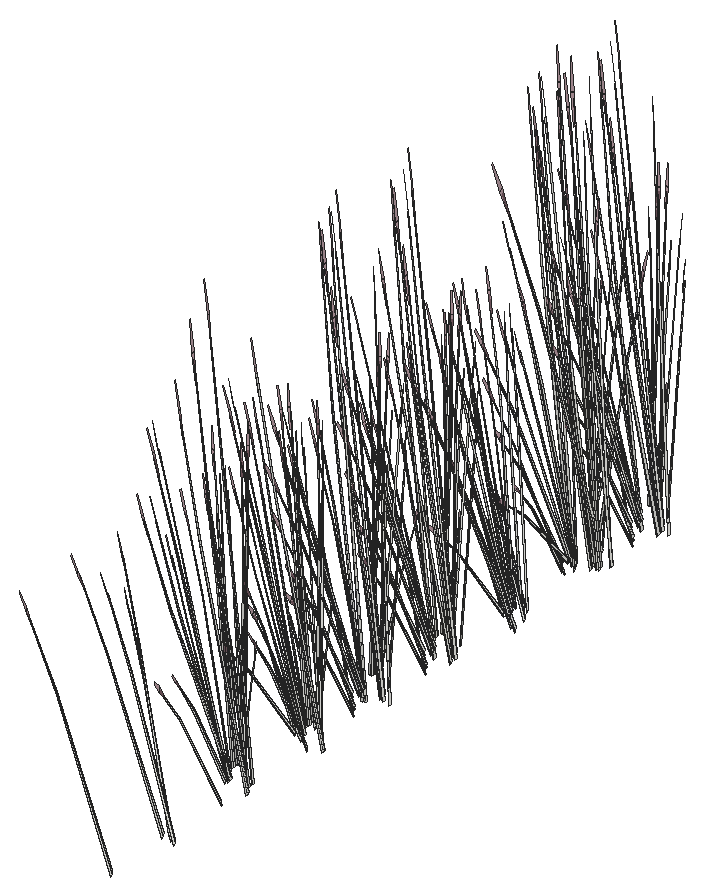
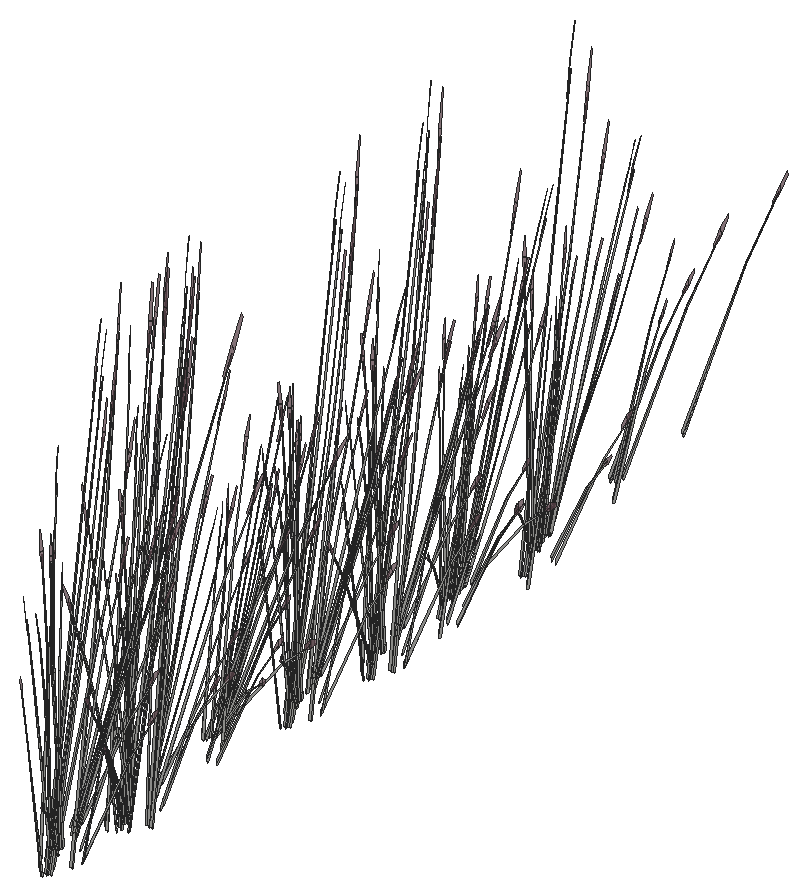
# SketchUp Ruby script. Lengths in inches.
U = 1.inch
M = Sketchup.active_model
def pt(a) = Geom::Point3d.new(a.map { |v| v * U })
def face(e, loops, mat)
  f = e.add_face(loops[0].map { |a| pt(a) })
  loops[1..].each { |l| e.add_face(l.map { |a| pt(a) }).erase! }
  f.material = f.back_material = mat if mat
  f
end
# faces: each face lists its corners as indices into pts; further lists are holes
def faces(e, pts, list, mat = nil) = list.each { |f| face(e, (f[0].is_a?(Array) ? f : [f]).map { |l| l.map { |i| pts[i] } }, mat) }
# xy, xz, yz: faces in a plane at the given z, y or x. An outline is a flat list of corners, or four numbers for a rectangle; further outlines are holes
def ring(l) = l.size == 4 ? [[l[0], l[1]], [l[2], l[1]], [l[2], l[3]], [l[0], l[3]]] : l.each_slice(2).to_a
def flat(e, list, mat, &to3) = list.each { |f| face(e, (f[0].is_a?(Array) ? f : [f]).map { |l| ring(l).map { |u, v| to3.(u, v) } }, mat) }
def xy(e, z, list, mat = nil) = flat(e, list, mat) { |x, y| [x, y, z] }
def xz(e, y, list, mat = nil) = flat(e, list, mat) { |x, z| [x, y, z] }
def yz(e, x, list, mat = nil) = flat(e, list, mat) { |y, z| [x, y, z] }
def lines(e, pts, list) = list.each { |a, b| e.add_line(pt(pts[a]), pt(pts[b])) }
# prism: a flat outline (further loops are holes) pulled along v
def prism(e, loops, v, mat = nil)
  f = face(e, loops, mat); d = Geom::Vector3d.new(v.map { |x| x * U })
  f.pushpull(f.normal.samedirection?(d) ? d.length : -d.length)
end
def box(e, o, s, mat = nil) = prism(e, [[o, [o[0] + s[0], o[1], o[2]], [o[0] + s[0], o[1] + s[1], o[2]], [o[0], o[1] + s[1], o[2]]]], [0, 0, s[2]], mat)
def at(x, y, z, deg = 0) = Geom::Transformation.translation(pt([x, y, z])) * Geom::Transformation.rotation(ORIGIN, Z_AXIS, deg.degrees)
def axes(o, x, y, z) = Geom::Transformation.new([*x, 0, *y, 0, *z, 0, *pt(o).to_a, 1])
def part(name) = M.definitions.add(name)
# library, detail: a bought-in or finely detailed component or shape, given as its bounding box
def library(name, o, s) = part(name).tap { |d| box(d.entities, o, s) }
def detail(e, o, s) = box(e.add_group.entities, o, s)
def put(e, d, t, mat = nil) = e.add_instance(d, t).tap { |i| i.material = mat if mat }
def group(e, t, mat = nil) = e.add_group.tap { |g| g.transformation = t; g.material = mat if mat }.entities
root = M.entities
M.materials.add("LightPink_Translucent").color = [144, 107, 117]
M.materials["LightPink_Translucent"].alpha = 0.75
c1 = part("blade")
p = [[2.15,0.21,22],[0,0.17,0],[0.09,0.45,0],[2.18,0.31,22],[2.29,0.31,22],[0.38,0.45,0],
  [2.48,0.24,33],[2.49,0.24,33],[2.48,0.22,33]]
faces(c1.entities,p,[[0,1,2,3],[4,5,2,3],[6,3,4,7],[8,0,3,6]])
c2 = part("seeds")
p = [[0.3,-0.1,1.38],[-0.01,-0.03,1.59],[-0.01,-0.03,0.03],[0.14,-0.07,-0.07],[0.29,-0.03,3],[0.15,0.01,3.11]]
faces(c2.entities,p,[[0,1,2,3],[1,0,4,5]],"LightPink_Translucent")
c3 = part("blade with seeds")
put(c3.entities,c1,at(0,0,0))
put(c3.entities,c2,axes([2.4,0.25,30.99],[1.5799,-0.05474,1.17369],[-0.12525,1.92788,0.29478],[-0.07173,-0.02425,1.56792]))
put(root,c3,axes([401.41,385.93,-7.3],[0.42502,0.15163,0.32977],[-0.12396,0.44238,-0.42575],[-0.17112,0.04056,0.81462]))
put(root,c3,axes([402.65,354.11,-8.39],[0.12773,-0.16701,1.59586],[0.32252,0.4508,0.12904],[-0.22121,0.20529,0.68222]))
put(root,c3,axes([402.3,364.67,-10.61],[0.01297,0.08566,1.6421],[-0.26146,0.44735,-0.25086],[-0.18572,-0.02255,0.2797]))
put(root,c3,axes([401.6,374.12,-7.3],[0.29098,0.34031,0.32977],[-0.33226,0.32215,-0.42575],[-0.16881,-0.04902,0.81462]))
put(root,c3,axes([401.49,417.08,-7.6],[0.02575,-0.41332,0.05988],[0.38885,0.01133,0.47138],[-0.14895,-0.04325,0.71878]))
put(root,c3,axes([401.88,354.55,-7.78],[-0.44516,0.07768,-0.32977],[-0.11755,-0.44407,0.42575],[-0.12757,0.11927,0.81462]))
put(root,c3,axes([400.57,420.61,-7.61],[-0.01271,0.10756,1.62908],[0.36076,0.37419,-0.25764],[-0.09444,0.17695,0.13065]))
put(root,c3,axes([402.39,373.52,-7.36],[-0.43608,-0.26272,-0.66157],[0.30991,-0.46038,0.07984],[-0.158,-0.15687,0.93586]))
put(root,c3,axes([402.59,419.37,-10.08],[-0.53199,-0.08911,-0.58063],[0.11226,-0.54969,-0.15239],[-0.15876,-0.06661,1.28164]))
put(root,c3,axes([402.68,416.37,-6.94],[-0.34131,0.52108,-0.12682],[-0.49429,-0.3002,-0.70393],[-0.17182,-0.14722,1.06961]))
put(root,c3,axes([401.6,405.53,-7.62],[-0.00954,0.06515,1.65179],[-0.47055,0.23645,-0.15608],[-0.13847,-0.12087,0.29231]))
put(root,c3,axes([402.18,373.53,-7.64],[-0.50465,0.12921,-0.47583],[-0.08828,-0.48932,-0.36857],[-0.13555,-0.14022,0.91046]))
put(root,c3,axes([401.48,387.31,-7.64],[0.13138,0.49631,-0.47583],[-0.49754,0.08682,-0.36857],[-0.14258,0.13331,0.91046]))
put(root,c3,axes([401.64,355.87,-10.61],[0.0686,0.0543,1.6421],[0.11632,0.50315,-0.25086],[-0.15204,0.10729,0.2797]))
put(root,c3,axes([402.37,362.625,-7.62],[0.03791,0.05424,1.65179],[-0.18278,0.48761,-0.15608],[-0.18511,0.00353,0.29231]))
put(root,c3,axes([401.62,384.67,-7.6],[0.02575,-0.41332,0.05988],[0.38885,0.01133,0.47138],[-0.14895,-0.04325,0.71878]))
put(root,c3,axes([401.1,406.47,-9.59],[-0.03097,0.17781,1.33163],[-0.45273,0.14885,-0.28638],[-0.10583,-0.22982,0.56934]))
put(root,c3,axes([401.75,417.39,-7.3],[0.29098,0.34031,0.32977],[-0.33226,0.32215,-0.42575],[-0.16881,-0.04902,0.81462]))
put(root,c3,axes([400.7,388.2,-7.61],[-0.01271,0.10756,1.62908],[0.36076,0.37419,-0.25764],[-0.09444,0.17695,0.13065]))
put(root,c3,axes([401.54,352.91,-9.42],[0.3265,-0.03889,1.06958],[-0.20711,0.3427,0.78586],[-0.16135,-0.05141,0.23558]))
put(root,c3,axes([404.56,395.59,-8.89],[0.14537,-0.07863,1.64882],[0.05013,0.549,0.12904],[-0.31487,0.07285,0.5893]))
put(root,c3,axes([401.24,406.93,-8.39],[0.1169,0.17452,1.59586],[-0.54019,0.14692,0.12904],[-0.12209,-0.27397,0.68222]))
put(root,c3,axes([402.72,386.95,-10.08],[-0.53199,-0.08911,-0.58063],[0.11226,-0.54969,-0.15239],[-0.15876,-0.06661,1.28164]))
put(root,c3,axes([402.53,416.79,-7.36],[-0.43608,-0.26272,-0.66157],[0.30991,-0.46038,0.07984],[-0.158,-0.15687,0.93586]))
put(root,c3,axes([402.82,383.95,-6.94],[-0.34131,0.52108,-0.12682],[-0.49429,-0.3002,-0.70393],[-0.17182,-0.14722,1.06961]))
put(root,c3,axes([402.24,409.85,-9.52],[-0.51635,0.36087,-0.27094],[-0.34336,-0.5099,-0.46562],[-0.1274,-0.05178,1.4872]))
put(root,c3,axes([402.33,416.8,-7.64],[-0.50465,0.12921,-0.47583],[-0.08828,-0.48932,-0.36857],[-0.13555,-0.14022,0.91046]))
put(root,c3,axes([401.6,366.82,-9.42],[0.21313,-0.24635,1.06958],[0.0841,0.38999,0.78586],[-0.15402,0.06983,0.23558]))
put(root,c3,axes([401.74,377.13,-10.12],[-0.47863,-0.27177,-0.46235],[0.28609,-0.48733,0],[-0.10901,-0.0619,1.46668]))
put(root,c3,axes([400.8125,410.98,-7.59],[-0.36417,-0.37086,0.447],[0.38674,-0.31985,0.36857],[-0.06718,0.174,0.92496]))
put(root,c3,axes([401.53,373.08,-10.61],[-0.04954,0.0716,1.6421],[-0.50062,0.15438,-0.25086],[-0.12094,-0.14044,0.2797]))
put(root,c3,axes([400.97,376.09,-7.3125],[0.47307,0.29971,-0.11324],[-0.27254,0.43404,-0.62851],[-0.13365,0.15087,0.95501]))
put(root,c3,axes([402.79,362.3,-7.61],[-0.11004,-0.00384,1.62908],[-0.35032,0.38367,-0.25764],[-0.18692,-0.07839,0.13065]))
put(root,c3,axes([401.88,384.98,-7.3],[0.29098,0.34031,0.32977],[-0.33226,0.32215,-0.42575],[-0.16881,-0.04902,0.81462]))
put(root,c3,axes([401.94,354.45,-7.59],[-0.12683,-0.50025,0.447],[0.49754,-0.08682,0.36857],[-0.14663,0.11765,0.92496]))
put(root,c3,axes([401.43,406.84,-7.78],[-0.07899,-0.43781,-0.32977],[0.45153,-0.11561,0.42575],[-0.12128,-0.12546,0.81462]))
put(root,c3,axes([402.67,384.375,-7.36],[-0.43608,-0.26272,-0.66157],[0.30991,-0.46038,0.07984],[-0.158,-0.15687,0.93586]))
put(root,c3,axes([400.17,409.06,-9.79],[-0.63949,0,0],[0,-0.60749,-0.48057],[0,-0.13836,1.52448]))
put(root,c3,axes([401.07,410.6,-10.11],[-0.12013,-0.47362,-0.28847],[0.47712,-0.13449,0.28847],[-0.09619,-0.05462,1.29413]))
put(root,c3,axes([402.03,377.46,-9.79],[-0.31974,0.54466,0],[-0.53494,-0.30375,-0.48057],[-0.12184,-0.06918,1.52448]))
put(root,c3,axes([402.46,384.39,-7.64],[-0.50465,0.12921,-0.47583],[-0.08828,-0.48932,-0.36857],[-0.13555,-0.14022,0.91046]))
put(root,c3,axes([402.34,364.42,-7.59],[0.14449,-0.4956,0.447],[0.47502,0.16947,0.36857],[-0.1868,0.02978,0.92496]))
put(root,c3,axes([400.68,410.95,-7.6],[-0.42027,-0.02533,0.05988],[0.01152,-0.38243,0.47138],[-0.04398,0.14649,0.71878]))
put(root,c3,axes([401.89,420.41,-10.12],[-0.47863,-0.27177,-0.46235],[0.28609,-0.48733,0],[-0.10901,-0.0619,1.46668]))
put(root,c3,axes([402.2,351.96,-7.26],[0.42234,-0.40113,0.50064],[0.36424,0.42599,0.4128],[-0.19815,-0.07399,1.03595]))
put(root,c3,axes([402.51,364.28,-7.3125],[0.25732,0.49218,-0.11324],[-0.45669,0.24187,-0.62851],[-0.19245,0.06494,0.95501]))
put(root,c3,axes([401.68,416.36,-10.61],[-0.04954,0.0716,1.6421],[-0.50062,0.15438,-0.25086],[-0.12094,-0.14044,0.2797]))
put(root,c3,axes([401.11,419.37,-7.3125],[0.47307,0.29971,-0.11324],[-0.27254,0.43404,-0.62851],[-0.13365,0.15087,0.95501]))
put(root,c3,axes([403.09,363.26,-7.3125],[-0.02738,0.55277,-0.11324],[-0.51847,-0.01511,-0.62851],[-0.19968,-0.0384,0.95501]))
put(root,c3,axes([401.84,354.36,-7.6],[-0.35109,-0.22859,0.05988],[0.2044,-0.32553,0.47138],[-0.11256,0.10524,0.71878]))
put(root,c3,axes([400.8125,411.1,-7.78],[-0.34603,0.28618,-0.32977],[-0.32756,-0.32677,0.42575],[-0.04984,0.16603,0.81462]))
put(root,c3,axes([402.76,363.3,-7.78],[-0.29098,-0.34031,-0.32977],[0.33226,-0.32215,0.42575],[-0.16881,-0.04902,0.81462]))
put(root,c3,axes([402.31,364.29,-7.6],[-0.18783,-0.37061,0.05988],[0.34252,-0.1814,0.47138],[-0.15099,0.03579,0.71878]))
put(root,c3,axes([404.59,339.29,-8.39],[0.21212,-0.01231,1.59586],[-0.14072,0.53355,0.12904],[-0.3023,-0.033,0.68222]))
put(root,c3,axes([402.18,420.73,-9.79],[-0.31974,0.54466,0],[-0.53494,-0.30375,-0.48057],[-0.12184,-0.06918,1.52448]))
put(root,c3,axes([403,395.96,-7.61],[-0.08351,0.07057,1.62908],[0.0071,0.51561,-0.25764],[-0.19143,0.06705,0.13065]))
put(root,c3,axes([403.17,365.32,-8.39],[0.12773,-0.16701,1.59586],[0.32252,0.4508,0.12904],[-0.22121,0.20529,0.68222]))
put(root,c3,axes([402.02,387.99,-10.12],[-0.47863,-0.27177,-0.46235],[0.28609,-0.48733,0],[-0.10901,-0.0619,1.46668]))
put(root,c3,axes([402.4,365.75,-7.78],[-0.44516,0.07768,-0.32977],[-0.11755,-0.44407,0.42575],[-0.12757,0.11927,0.81462]))
put(root,c3,axes([404.08,394.71,-7.36],[-0.51122,-0.01309,-0.66157],[0.03434,-0.5511,0.07984],[-0.21658,-0.05816,0.93586]))
put(root,c3,axes([401.8125,383.94,-10.61],[-0.04954,0.0716,1.6421],[-0.50062,0.15438,-0.25086],[-0.12094,-0.14044,0.2797]))
put(root,c3,axes([401.25,386.95,-7.3125],[0.47307,0.29971,-0.11324],[-0.27254,0.43404,-0.62851],[-0.13365,0.15087,0.95501]))
put(root,c3,axes([400.1875,377.39,-6.74],[0.45129,0.14509,-0.06041],[-0.13882,0.44656,-0.27392],[-0.07381,0.0678,0.90349]))
put(root,c3,axes([403.67,394.84,-9.59],[0.09985,0.15133,1.33163],[-0.23008,0.41134,-0.28638],[-0.23625,-0.09832,0.56934]))
put(root,c3,axes([402.58,410.24,-10.08],[-0.34446,0.40855,-0.58063],[-0.42791,-0.37046,-0.15239],[-0.13803,0.10191,1.28164]))
put(root,c3,axes([402.56,354.52,-8.39],[0.09522,-0.18683,1.59586],[0.39947,0.38663,0.12904],[-0.18021,0.24097,0.68222]))
put(root,c3,axes([401.7,407.2,-7.3],[0.07899,0.43781,0.32977],[-0.45153,0.11561,-0.42575],[-0.12128,-0.12546,0.81462]))
put(root,c3,axes([402.16,367.07,-10.61],[0.0686,0.0543,1.6421],[0.11632,0.50315,-0.25086],[-0.15204,0.10729,0.2797]))
put(root,c3,axes([402.31,388.32,-9.79],[-0.31974,0.54466,0],[-0.53494,-0.30375,-0.48057],[-0.12184,-0.06918,1.52448]))
put(root,c3,axes([401.2,376.13,-7.3],[0.44516,-0.07768,0.32977],[0.11755,0.44407,-0.42575],[-0.12757,0.11927,0.81462]))
put(root,c3,axes([399.58,412.11,-7.62],[0.05802,-0.03282,1.65179],[0.47954,0.21828,-0.15608],[-0.01127,0.18175,0.29231]))
put(root,c3,axes([402.06,364.11,-9.42],[0.3265,-0.03889,1.06958],[-0.20711,0.3427,0.78586],[-0.16135,-0.05141,0.23558]))
put(root,c3,axes([403.26,395.66,-7.78],[-0.42502,-0.15163,-0.32977],[0.12396,-0.44238,0.42575],[-0.17112,0.04056,0.81462]))
put(root,c3,axes([400.67,408.9,-9.83],[-0.47569,0.45698,0.2864],[-0.47598,-0.45217,-0.33981],[-0.01661,-0.12977,1.53541]))
put(root,c3,axes([403.85,394.35,-8.39],[0.18996,0.09365,1.59586],[-0.39312,0.39287,0.12904],[-0.24502,-0.17723,0.68222]))
put(root,c3,axes([400.33,420.67,-6.74],[0.45129,0.14509,-0.06041],[-0.13882,0.44656,-0.27392],[-0.07381,0.0678,0.90349]))
put(root,c3,axes([401.45,378.25,-9.59],[0.16138,-0.08575,1.33163],[0.39845,0.25854,-0.28638],[-0.1186,0.22371,0.56934]))
put(root,c3,axes([402.63,410.16,-8.9],[0.44194,0.21918,1.40854],[-0.43295,0.47219,0.557],[-0.19393,-0.27986,1.18082]))
put(root,c3,axes([402.18,353.22,-7.3],[0.42502,0.15163,0.32977],[-0.12396,0.44238,-0.42575],[-0.17112,0.04056,0.81462]))
put(root,c3,axes([401.22,373.36,-10.02],[-0.14753,0.44383,-0.03625],[-0.45406,-0.13653,-0.16435],[-0.06894,-0.07259,0.54209]))
put(root,c3,axes([401.34,419.41,-7.3],[0.44516,-0.07768,0.32977],[0.11755,0.44407,-0.42575],[-0.12757,0.11927,0.81462]))
put(root,c3,axes([402.46,365.66,-7.59],[-0.12683,-0.50025,0.447],[0.49754,-0.08682,0.36857],[-0.14663,0.11765,0.92496]))
put(root,c3,axes([400.94,406.1875,-9.42],[0.26677,0.18918,1.06958],[-0.38851,0.11372,0.78586],[-0.08313,-0.14539,0.23558]))
put(root,c3,axes([402.82,410.01,-9.7],[-0.49938,-0.43748,-0.23459],[0.42021,-0.49126,0.51337],[-0.13447,0.05118,1.56642]))
put(root,c3,axes([400.47,388.25,-6.74],[0.45129,0.14509,-0.06041],[-0.13882,0.44656,-0.27392],[-0.07381,0.0678,0.90349]))
put(root,c3,axes([402.25,354.6,-7.64],[0.13138,0.49631,-0.47583],[-0.49754,0.08682,-0.36857],[-0.14258,0.13331,0.91046]))
put(root,c3,axes([401.6,421.52,-9.59],[0.16138,-0.08575,1.33163],[0.39845,0.25854,-0.28638],[-0.1186,0.22371,0.56934]))
put(root,c3,axes([401.91,409.59,-9.94],[-0.30722,-0.45622,-0.41661],[0.46535,-0.32126,0.2005],[-0.09942,-0.05645,1.33761]))
put(root,c3,axes([402.07,396.48,-7.62],[0.06527,0.01458,1.65179],[0.20191,0.48025,-0.15608],[-0.1336,0.12605,0.29231]))
put(root,c3,axes([402.4,371.85,-7.62],[-0.00954,0.06515,1.65179],[-0.47055,0.23645,-0.15608],[-0.13847,-0.12087,0.29231]))
put(root,c3,axes([403.56,395.89,-7.64],[-0.13855,0.49442,-0.47583],[-0.47502,-0.16947,-0.36857],[-0.19125,0.04534,0.91046]))
put(root,c3,axes([402.71,363.17,-7.26],[0.42234,-0.40113,0.50064],[0.36424,0.42599,0.4128],[-0.19815,-0.07399,1.03595]))
put(root,c3,axes([402.39,351.96,-7.6],[0.02575,-0.41332,0.05988],[0.38885,0.01133,0.47138],[-0.14895,-0.04325,0.71878]))
put(root,c3,axes([401.37,416.63,-10.02],[-0.14753,0.44383,-0.03625],[-0.45406,-0.13653,-0.16435],[-0.06894,-0.07259,0.54209]))
put(root,c3,axes([401.47,355.49,-7.61],[-0.01271,0.10756,1.62908],[0.36076,0.37419,-0.25764],[-0.09444,0.17695,0.13065]))
put(root,c3,axes([401.48,386.99,-7.3],[0.44516,-0.07768,0.32977],[0.11755,0.44407,-0.42575],[-0.12757,0.11927,0.81462]))
put(root,c3,axes([401.04,410.79,-7.03],[-0.01331,0.50278,-0.73435],[-0.56035,-0.03377,0.08862],[-0.05914,0.213,1.03881]))
put(root,c3,axes([401.9,372.8,-9.59],[-0.03097,0.17781,1.33163],[-0.45273,0.14885,-0.28638],[-0.10583,-0.22982,0.56934]))
put(root,c3,axes([402.36,365.5625,-7.6],[-0.35109,-0.22859,0.05988],[0.2044,-0.32553,0.47138],[-0.11256,0.10524,0.71878]))
put(root,c3,axes([403.49,354.25,-10.08],[-0.53199,-0.08911,-0.58063],[0.11226,-0.54969,-0.15239],[-0.15876,-0.06661,1.28164]))
put(root,c3,axes([403.59,351.25,-6.94],[-0.34131,0.52108,-0.12682],[-0.49429,-0.3002,-0.70393],[-0.17182,-0.14722,1.06961]))
put(root,c3,axes([402.05,373.26,-8.39],[0.1169,0.17452,1.59586],[-0.54019,0.14692,0.12904],[-0.12209,-0.27397,0.68222]))
put(root,c3,axes([403.92,394.82,-7.64],[-0.37135,0.36005,-0.47583],[-0.32522,-0.38035,-0.36857],[-0.18868,-0.05478,0.91046]))
put(root,c3,axes([401.73,389.11,-9.59],[0.16138,-0.08575,1.33163],[0.39845,0.25854,-0.28638],[-0.1186,0.22371,0.56934]))
put(root,c3,axes([401.03,412.21,-9.42],[-0.01324,-0.32319,1.06958],[0.33072,0.23052,0.78586],[-0.06504,0.15405,0.23558]))
put(root,c3,axes([401.5,406.68,-7.26],[0.56969,-0.13971,0.50064],[0.09887,0.54803,0.4128],[-0.13398,-0.16152,1.03595]))
put(root,c3,axes([403.32,395.86,-10.61],[0.01297,0.08566,1.6421],[-0.26146,0.44735,-0.25086],[-0.18572,-0.02255,0.2797]))
put(root,c3,axes([403.04,376.17,-9.52],[-0.51635,0.36087,-0.27094],[-0.34336,-0.5099,-0.46562],[-0.1274,-0.05178,1.4872]))
put(root,c3,axes([404.68,340.22,-8.39],[0.17745,-0.11497,1.59586],[0.14939,0.53127,0.12904],[-0.27857,0.12007,0.68222]))
put(root,c3,axes([402.55,415.13,-7.62],[-0.00954,0.06515,1.65179],[-0.47055,0.23645,-0.15608],[-0.13847,-0.12087,0.29231]))
put(root,c3,axes([401.5,384.22,-10.02],[-0.14753,0.44383,-0.03625],[-0.45406,-0.13653,-0.16435],[-0.06894,-0.07259,0.54209]))
put(root,c3,axes([402.65,352.27,-7.3],[0.29098,0.34031,0.32977],[-0.33226,0.32215,-0.42575],[-0.16881,-0.04902,0.81462]))
put(root,c3,axes([402.57,409.92,-9.94],[-0.55535,0.03355,-0.41661],[-0.05022,-0.55698,0.2005],[-0.09942,0.05645,1.33761]))
put(root,c3,axes([401.62,377.3125,-7.59],[-0.36417,-0.37086,0.447],[0.38674,-0.31985,0.36857],[-0.06718,0.174,0.92496]))
put(root,c3,axes([402.05,416.07,-9.59],[-0.03097,0.17781,1.33163],[-0.45273,0.14885,-0.28638],[-0.10583,-0.22982,0.56934]))
put(root,c3,axes([403.4375,351.67,-7.36],[-0.43608,-0.26272,-0.66157],[0.30991,-0.46038,0.07984],[-0.158,-0.15687,0.93586]))
put(root,c3,axes([402.24,373.17,-7.78],[-0.07899,-0.43781,-0.32977],[0.45153,-0.11561,0.42575],[-0.12128,-0.12546,0.81462]))
put(root,c3,axes([403.07,365.73,-8.39],[0.09522,-0.18683,1.59586],[0.39947,0.38663,0.12904],[-0.18021,0.24097,0.68222]))
put(root,c3,axes([403.23,351.68,-7.64],[-0.50465,0.12921,-0.47583],[-0.08828,-0.48932,-0.36857],[-0.13555,-0.14022,0.91046]))
put(root,c3,axes([404.13,341.13,-9.59],[0.17773,0.04462,1.33163],[0.11455,0.45576,-0.28638],[-0.24142,0.08531,0.56934]))
put(root,c3,axes([402.19,416.53,-8.39],[0.1169,0.17452,1.59586],[-0.54019,0.14692,0.12904],[-0.12209,-0.27397,0.68222]))
put(root,c3,axes([400.98,375.39,-9.79],[-0.63949,0,0],[0,-0.60749,-0.48057],[0,-0.13836,1.52448]))
put(root,c3,axes([403.39,393.8125,-7.62],[0.03791,0.05424,1.65179],[-0.18278,0.48761,-0.15608],[-0.18511,0.00353,0.29231]))
put(root,c3,axes([401.875,376.93,-10.11],[-0.12013,-0.47362,-0.28847],[0.47712,-0.13449,0.28847],[-0.09619,-0.05462,1.29413]))
put(root,c3,axes([402.69,382.71,-7.62],[-0.00954,0.06515,1.65179],[-0.47055,0.23645,-0.15608],[-0.13847,-0.12087,0.29231]))
put(root,c3,axes([403.19,419.45,-9.52],[-0.51635,0.36087,-0.27094],[-0.34336,-0.5099,-0.46562],[-0.1274,-0.05178,1.4872]))
put(root,c3,axes([401.48,377.28,-7.6],[-0.42027,-0.02533,0.05988],[0.01152,-0.38243,0.47138],[-0.04398,0.14649,0.71878]))
put(root,c3,axes([401.63,406.8,-7.6],[0.23243,-0.34529,0.05988],[0.331,0.20103,0.47138],[-0.10701,-0.1107,0.71878]))
put(root,c3,axes([401.76,420.59,-7.59],[-0.36417,-0.37086,0.447],[0.38674,-0.31985,0.36857],[-0.06718,0.174,0.92496]))
put(root,c3,axes([402.18,383.66,-9.59],[-0.03097,0.17781,1.33163],[-0.45273,0.14885,-0.28638],[-0.10583,-0.22982,0.56934]))
put(root,c3,axes([401.62,377.42,-7.78],[-0.34603,0.28618,-0.32977],[-0.32756,-0.32677,0.42575],[-0.04984,0.16603,0.81462]))
put(root,c3,axes([402.62,398.01,-9.42],[0.21313,-0.24635,1.06958],[0.0841,0.38999,0.78586],[-0.15402,0.06983,0.23558]))
put(root,c3,axes([405.35,330.35,-8.39],[0.21212,-0.01231,1.59586],[-0.14072,0.53355,0.12904],[-0.3023,-0.033,0.68222]))
put(root,c3,axes([401.51,410.85,-9.69],[0.47863,0.27177,0.46235],[-0.28609,0.48733,0],[-0.10901,-0.0619,1.46668]))
put(root,c3,axes([402.38,416.44,-7.78],[-0.07899,-0.43781,-0.32977],[0.45153,-0.11561,0.42575],[-0.12128,-0.12546,0.81462]))
put(root,c3,axes([402.33,384.12,-8.39],[0.1169,0.17452,1.59586],[-0.54019,0.14692,0.12904],[-0.12209,-0.27397,0.68222]))
put(root,c3,axes([402.69,364.43,-7.3],[0.42502,0.15163,0.32977],[-0.12396,0.44238,-0.42575],[-0.17112,0.04056,0.81462]))
put(root,c3,axes([400.86,411.5,-8.87],[0.01124,-0.2806,1.43727],[0.50537,0.14821,0.19862],[-0.04379,0.29905,0.67868]))
put(root,c3,axes([402.79,355.29,-10.12],[-0.47863,-0.27177,-0.46235],[0.28609,-0.48733,0],[-0.10901,-0.0619,1.46668]))
put(root,c3,axes([403.8125,393.49,-7.61],[-0.11004,-0.00384,1.62908],[-0.35032,0.38367,-0.25764],[-0.18692,-0.07839,0.13065]))
put(root,c3,axes([401.125,418.66,-9.79],[-0.63949,0,0],[0,-0.60749,-0.48057],[0,-0.13836,1.52448]))
put(root,c3,axes([403.32,387.03,-9.52],[-0.51635,0.36087,-0.27094],[-0.34336,-0.5099,-0.46562],[-0.1274,-0.05178,1.4872]))
put(root,c3,axes([402.02,420.2,-10.11],[-0.12013,-0.47362,-0.28847],[0.47712,-0.13449,0.28847],[-0.09619,-0.05462,1.29413]))
put(root,c3,axes([405.7,339.67,-8.89],[0.14537,-0.07863,1.64882],[0.05013,0.549,0.12904],[-0.31487,0.07285,0.5893]))
put(root,c3,axes([402.58,351.24,-10.61],[-0.04954,0.0716,1.6421],[-0.50062,0.15438,-0.25086],[-0.12094,-0.14044,0.2797]))
put(root,c3,axes([402.02,354.25,-7.3125],[0.47307,0.29971,-0.11324],[-0.27254,0.43404,-0.62851],[-0.13365,0.15087,0.95501]))
put(root,c3,axes([401.63,420.55,-7.6],[-0.42027,-0.02533,0.05988],[0.01152,-0.38243,0.47138],[-0.04398,0.14649,0.71878]))
put(root,c3,axes([401.9,388.17,-7.59],[-0.36417,-0.37086,0.447],[0.38674,-0.31985,0.36857],[-0.06718,0.174,0.92496]))
put(root,c3,axes([401.96,409.85,-9.73],[0.13555,-0.64407,-0.21817],[0.64269,0.11227,0.47743],[-0.1123,-0.08895,1.45677]))
put(root,c3,axes([402.77,365.81,-7.64],[0.13138,0.49631,-0.47583],[-0.49754,0.08682,-0.36857],[-0.14258,0.13331,0.91046]))
put(root,c3,axes([403.36,395.61,-7.59],[0.14449,-0.4956,0.447],[0.47502,0.16947,0.36857],[-0.1868,0.02978,0.92496]))
put(root,c3,axes([401.76,420.7,-7.78],[-0.34603,0.28618,-0.32977],[-0.32756,-0.32677,0.42575],[-0.04984,0.16603,0.81462]))
put(root,c3,axes([402.52,384.03,-7.78],[-0.07899,-0.43781,-0.32977],[0.45153,-0.11561,0.42575],[-0.12128,-0.12546,0.81462]))
put(root,c3,axes([403.39,376.57,-10.08],[-0.34446,0.40855,-0.58063],[-0.42791,-0.37046,-0.15239],[-0.13803,0.10191,1.28164]))
put(root,c3,axes([403.08,355.61,-9.79],[-0.31974,0.54466,0],[-0.53494,-0.30375,-0.48057],[-0.12184,-0.06918,1.52448]))
put(root,c3,axes([403.53,395.47,-7.3125],[0.25732,0.49218,-0.11324],[-0.45669,0.24187,-0.62851],[-0.19245,0.06494,0.95501]))
put(root,c3,axes([402.91,363.17,-7.6],[0.02575,-0.41332,0.05988],[0.38885,0.01133,0.47138],[-0.14895,-0.04325,0.71878]))
put(root,c3,axes([402.5,373.53,-7.3],[0.07899,0.43781,0.32977],[-0.45153,0.11561,-0.42575],[-0.12128,-0.12546,0.81462]))
put(root,c3,axes([401.99,366.7,-7.61],[-0.01271,0.10756,1.62908],[0.36076,0.37419,-0.25764],[-0.09444,0.17695,0.13065]))
put(root,c3,axes([401.26,386.24,-9.79],[-0.63949,0,0],[0,-0.60749,-0.48057],[0,-0.13836,1.52448]))
put(root,c3,axes([402.16,387.79,-10.11],[-0.12013,-0.47362,-0.28847],[0.47712,-0.13449,0.28847],[-0.09619,-0.05462,1.29413]))
put(root,c3,axes([404.11,394.44,-7.3125],[-0.02738,0.55277,-0.11324],[-0.51847,-0.01511,-0.62851],[-0.19968,-0.0384,0.95501]))
put(root,c3,axes([402.19,410,-9.5625],[-0.09866,0.48509,0.13483],[-0.48202,-0.0842,-0.38503],[-0.08772,-0.04981,1.18024]))
put(root,c3,axes([400.38,378.44,-7.62],[0.05802,-0.03282,1.65179],[0.47954,0.21828,-0.15608],[-0.01127,0.18175,0.29231]))
put(root,c3,axes([401.76,388.14,-7.6],[-0.42027,-0.02533,0.05988],[0.01152,-0.38243,0.47138],[-0.04398,0.14649,0.71878]))
put(root,c3,axes([403.78,394.48,-7.78],[-0.29098,-0.34031,-0.32977],[0.33226,-0.32215,0.42575],[-0.16881,-0.04902,0.81462]))
put(root,c3,axes([404.01,365.45,-10.08],[-0.53199,-0.08911,-0.58063],[0.11226,-0.54969,-0.15239],[-0.15876,-0.06661,1.28164]))
put(root,c3,axes([401.47,375.23,-9.83],[-0.47569,0.45698,0.2864],[-0.47598,-0.45217,-0.33981],[-0.01661,-0.12977,1.53541]))
put(root,c3,axes([403.33,395.48,-7.6],[-0.18783,-0.37061,0.05988],[0.34252,-0.1814,0.47138],[-0.15099,0.03579,0.71878]))
put(root,c3,axes([404.1,362.45,-6.94],[-0.34131,0.52108,-0.12682],[-0.49429,-0.3002,-0.70393],[-0.17182,-0.14722,1.06961]))
put(root,c3,axes([402.14,405.78,-7.61],[-0.07822,-0.07621,1.62908],[-0.52201,0.04832,-0.25764],[-0.08331,-0.18228,0.13065]))
put(root,c3,axes([403.15,411.35,-10.12],[-0.47863,0.27177,-0.46235],[-0.28609,-0.48733,0],[-0.10901,0.0619,1.46668]))
put(root,c3,axes([401.9,388.28,-7.78],[-0.34603,0.28618,-0.32977],[-0.32756,-0.32677,0.42575],[-0.04984,0.16603,0.81462]))
put(root,c3,axes([404.1875,396.5,-8.39],[0.12773,-0.16701,1.59586],[0.32252,0.4508,0.12904],[-0.22121,0.20529,0.68222]))
put(root,c3,axes([400.32,408.65,-10.12],[0,-0.54355,-0.46235],[0.57217,0,0],[0,-0.1238,1.46668]))
put(root,c3,axes([403.42,396.94,-7.78],[-0.44516,0.07768,-0.32977],[-0.11755,-0.44407,0.42575],[-0.12757,0.11927,0.81462]))
put(root,c3,axes([400.5625,409.15,-9.69],[0,0.54355,0.46235],[-0.57217,0,0],[0,-0.1238,1.46668]))
put(root,c3,axes([403.53,419.84,-10.08],[-0.34446,0.40855,-0.58063],[-0.42791,-0.37046,-0.15239],[-0.13803,0.10191,1.28164]))
put(root,c3,axes([403.18,411.21,-9.96],[-0.31576,-0.54657,-0.04789],[0.53494,-0.30375,0.48057],[-0.13182,0.05204,1.52373]))
